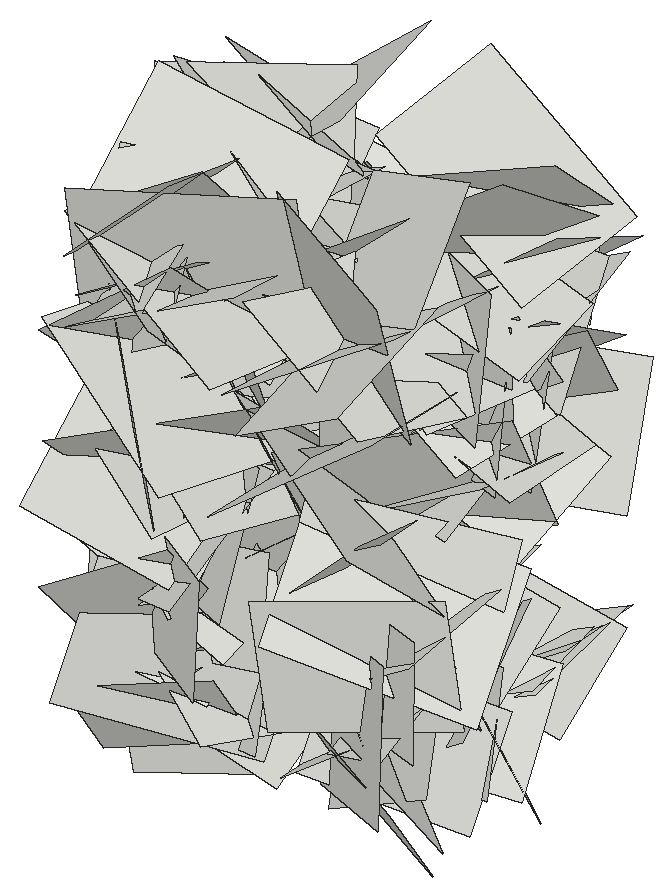
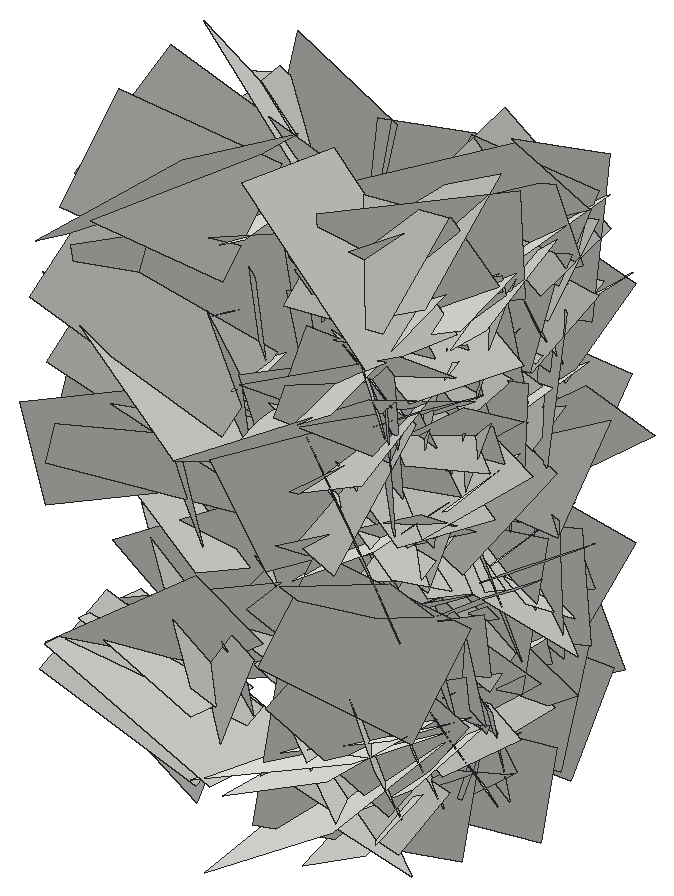
# SketchUp Ruby script. Lengths in inches.
U = 1.inch
M = Sketchup.active_model
def pt(a) = Geom::Point3d.new(a.map { |v| v * U })
def face(e, loops, mat)
  f = e.add_face(loops[0].map { |a| pt(a) })
  loops[1..].each { |l| e.add_face(l.map { |a| pt(a) }).erase! }
  f.material = f.back_material = mat if mat
  f
end
# faces: each face lists its corners as indices into pts; further lists are holes
def faces(e, pts, list, mat = nil) = list.each { |f| face(e, (f[0].is_a?(Array) ? f : [f]).map { |l| l.map { |i| pts[i] } }, mat) }
# xy, xz, yz: faces in a plane at the given z, y or x. An outline is a flat list of corners, or four numbers for a rectangle; further outlines are holes
def ring(l) = l.size == 4 ? [[l[0], l[1]], [l[2], l[1]], [l[2], l[3]], [l[0], l[3]]] : l.each_slice(2).to_a
def flat(e, list, mat, &to3) = list.each { |f| face(e, (f[0].is_a?(Array) ? f : [f]).map { |l| ring(l).map { |u, v| to3.(u, v) } }, mat) }
def xy(e, z, list, mat = nil) = flat(e, list, mat) { |x, y| [x, y, z] }
def xz(e, y, list, mat = nil) = flat(e, list, mat) { |x, z| [x, y, z] }
def yz(e, x, list, mat = nil) = flat(e, list, mat) { |y, z| [x, y, z] }
def lines(e, pts, list) = list.each { |a, b| e.add_line(pt(pts[a]), pt(pts[b])) }
# prism: a flat outline (further loops are holes) pulled along v
def prism(e, loops, v, mat = nil)
  f = face(e, loops, mat); d = Geom::Vector3d.new(v.map { |x| x * U })
  f.pushpull(f.normal.samedirection?(d) ? d.length : -d.length)
end
def box(e, o, s, mat = nil) = prism(e, [[o, [o[0] + s[0], o[1], o[2]], [o[0] + s[0], o[1] + s[1], o[2]], [o[0], o[1] + s[1], o[2]]]], [0, 0, s[2]], mat)
def at(x, y, z, deg = 0) = Geom::Transformation.translation(pt([x, y, z])) * Geom::Transformation.rotation(ORIGIN, Z_AXIS, deg.degrees)
def axes(o, x, y, z) = Geom::Transformation.new([*x, 0, *y, 0, *z, 0, *pt(o).to_a, 1])
def part(name) = M.definitions.add(name)
# library, detail: a bought-in or finely detailed component or shape, given as its bounding box
def library(name, o, s) = part(name).tap { |d| box(d.entities, o, s) }
def detail(e, o, s) = box(e.add_group.entities, o, s)
def put(e, d, t, mat = nil) = e.add_instance(d, t).tap { |i| i.material = mat if mat }
def group(e, t, mat = nil) = e.add_group.tap { |g| g.transformation = t; g.material = mat if mat }.entities
root = M.entities
c1 = part("Component\#6")
p = [[0.01,0,0],[0,3.24,4.54],[4.32,3.24,4.54],[4.33,0,0]]
faces(c1.entities,p,[[0,1,2,3]])
put(root,c1,axes([414.68,192.1875,23.6],[-0.04344,0.89705,-0.17333],[0.1764,-0.16328,-0.88435],[-0.95226,-0.07116,-0.15591]))
put(root,c1,axes([410.71,200.85,9.74],[0.02518,0.49854,0.49521],[0.19267,0.47427,-0.48618],[0.7195,-0.14445,0.11286]))
put(root,c1,axes([414.68,200.46,4.14],[-0.03987,0.66432,-0.22968],[-0.12809,-0.2327,-0.65325],[-0.73398,0.00452,0.12648]))
put(root,c1,axes([410.71,196.11,19.5625],[-0.1708,0.27531,1.11719],[-0.21419,1.10379,-0.30115],[1.2007,0.23607,0.1052]))
put(root,c1,axes([410.71,195.27,-1.16],[-0.10176,-0.07093,0.82892],[0.16666,0.81783,0.08819],[0.86597,-0.16573,0.08043]))
put(root,c1,axes([414.68,202.11,15.27],[-0.00741,-0.76642,-0.19435],[-0.02033,-0.19414,0.76626],[-0.83787,0.01149,-0.01688]))
put(root,c1,axes([414.68,201.99,11.3125],[0.07595,0.62186,-0.76254],[0.14567,-0.76339,-0.60964],[-1.03278,-0.06194,-0.14206]))
put(root,c1,axes([410.71,202.38,16.09],[-0.07402,-0.92988,-0.45649],[-0.17154,-0.44211,0.92536],[1.08456,-0.13339,0.1152]))
put(root,c1,axes([410.71,193.92,18.08],[-0.13809,0.41624,-1.10581],[-0.27382,-1.09563,-0.38198],[1.22215,-0.19844,-0.21052]))
put(root,c1,axes([414.68,193.9,23.36],[-0.05376,0.55183,-0.55937],[0.04326,-0.55793,-0.55411],[-0.83178,-0.06469,0.00734]))
put(root,c1,axes([410.71,196.25,20.97],[0.03433,0.46285,-0.75346],[-0.09275,-0.74858,-0.46362],[0.93272,-0.09148,-0.01837]))
put(root,c1,axes([410.71,193.09,19.46],[0.07295,0.25641,0.83596],[-0.12348,0.83376,-0.24615],[0.9186,0.09171,-0.09948]))
put(root,c1,axes([414.68,200.69,6.875],[0.16125,-0.91938,-0.30199],[0.04119,-0.29965,0.93182],[-1.02494,-0.15668,-0.01006]))
put(root,c1,axes([410.71,194.43,21.03],[-0.18864,1.08922,-0.2367],[-0.12278,-0.25647,-1.09312],[1.17512,0.14806,-0.15221]))
put(root,c1,axes([410.71,195.95,14.86],[-0.17446,0.9838,0.62037],[-0.19333,0.59697,-0.99508],[1.2176,0.23574,-0.06911]))
put(root,c1,axes([410.71,200.41,3.58],[-0.05776,-0.87144,-0.04483],[0.06577,-0.04867,0.87073],[0.92261,-0.05109,-0.06488]))
put(root,c1,axes([410.71,198.3125,4.47],[-0.08144,0.93817,-0.09306],[-0.01009,-0.09413,-0.94116],[0.99929,0.07551,-0.01709]))
put(root,c1,axes([410.71,200.05,13.66],[0.07814,0.81604,-0.08962],[-0.02759,-0.08761,-0.81916],[0.86976,-0.0761,-0.01794]))
put(root,c1,axes([410.71,196.375,20.79],[-0.12547,0.87042,-0.10702],[0.18806,-0.08199,-0.86307],[0.91037,0.1369,0.16354]))
put(root,c1,axes([410.71,195.73,16.63],[-0.01219,-0.78698,0.32297],[0.05977,0.32158,0.78561],[0.89973,-0.03203,-0.04781]))
put(root,c1,axes([414.68,200.82,0.59],[-0.02153,-0.73416,-0.35765],[0.0933,-0.35764,0.72915],[-0.8606,-0.02041,0.08799]))
put(root,c1,axes([410.71,193.46,10.77],[0.10152,0.90556,-0.18731],[-0.17799,-0.16815,-0.89879],[0.96391,-0.12642,-0.14624]))
put(root,c1,axes([410.71,196.17,12.88],[-0.06274,0.02618,0.84664],[0.15393,0.83645,-0.01571],[0.88457,-0.1437,0.06278]))
put(root,c1,axes([410.71,195.4375,18.11],[0.16874,-0.51977,-0.57708],[-0.05885,-0.59519,0.52076],[0.82114,0.06415,0.15591]))
put(root,c1,axes([414.68,195.9375,9.16],[-0.07841,0.69576,-0.29748],[0.09095,-0.28926,-0.69787],[-0.79692,-0.10147,-0.05038]))
put(root,c1,axes([410.71,198.67,11.97],[-0.07539,0.76068,0.50866],[0.0723,0.51318,-0.75791],[0.96729,0.02092,0.0963]))
put(root,c1,axes([414.68,195.99,4.23],[0.18601,0.0566,0.88651],[-0.05201,0.90288,-0.04793],[-0.94017,-0.03875,0.17804]))
put(root,c1,axes([414.68,197.35,3.52],[-0.03443,0.41092,0.66217],[0.08038,0.66126,-0.40665],[-0.82215,0.04744,-0.06748]))
put(root,c1,axes([410.71,192.22,20.81],[0.00161,0.62306,-0.59539],[0.0785,-0.59329,-0.62067],[0.91013,0.05007,0.05459]))
put(root,c1,axes([414.68,202.74,-0.14],[-0.03158,-0.64507,0.25861],[-0.01592,0.25938,0.64528],[-0.73651,0.02205,-0.02503]))
put(root,c1,axes([410.71,195.86,16.68],[0.06531,-0.43873,0.684],[0.07025,0.68639,0.43429],[0.8585,-0.02279,-0.08757]))
put(root,c1,axes([414.68,202.51,19.98],[-0.06792,0.48446,-0.5602],[0.10116,-0.55221,-0.48846],[-0.77852,-0.11402,-0.01459]))
put(root,c1,axes([414.68,192.04,10.01],[0.12172,0.5206,-0.6372],[-0.01939,-0.6416,-0.52749],[-0.87198,0.08694,-0.07722]))
put(root,c1,axes([414.68,198.38,4.95],[0.02223,0.32868,-0.55446],[-0.17267,-0.53404,-0.32274],[-0.66105,0.15055,0.06565]))
put(root,c1,axes([410.71,199.37,10.67],[-0.09558,-1.01864,0.46326],[-0.13943,0.47118,1.01047],[1.17795,-0.02688,0.1572]))
put(root,c1,axes([414.68,192.95,10.8],[-0.02962,0.02518,0.78508],[0.12702,0.77652,-0.02064],[-0.82287,0.11896,-0.03145]))
put(root,c1,axes([414.68,200.03,9.27],[0.00412,-0.60297,0.30435],[-0.07057,0.30253,0.60022],[-0.71247,-0.03345,-0.05769]))
put(root,c1,axes([414.68,199.6875,17.84],[-0.07891,0.44569,0.39814],[-0.07493,0.39183,-0.45185],[-0.62903,-0.10259,0.00388]))
put(root,c1,axes([414.68,200.4375,8.06],[0.17377,0.75884,-0.49804],[0.05898,-0.51355,-0.76415],[-0.96033,0.10576,-0.13705]))
put(root,c1,axes([414.68,195.68,15.75],[-0.06715,-0.51242,0.33521],[-0.05381,0.34023,0.51051],[-0.64683,0.02489,-0.07727]))
put(root,c1,axes([414.68,198.91,12.75],[0.15355,-0.10183,1.00426],[0.21738,0.99636,0.07145],[-1.04766,0.19182,0.16201]))
put(root,c1,axes([414.68,196.5625,6.92],[-0.07674,-0.09799,-0.6482],[0.03176,-0.65195,0.09521],[-0.69417,-0.019,0.07601]))
put(root,c1,axes([414.68,199.23,1.1],[0.00098,-0.71414,-0.15761],[0.04174,-0.15733,0.71311],[-0.77408,-0.00939,0.03826]))
put(root,c1,axes([414.68,192.26,20.51],[0.14395,0.6641,-0.62024],[0.10915,-0.63433,-0.65665],[-0.95701,0.02754,-0.16819]))
put(root,c1,axes([414.68,193.91,15.9375],[-0.03263,0.61645,-0.26034],[0.02336,-0.25954,-0.61716],[-0.70894,-0.03692,-0.00835]))
put(root,c1,axes([414.68,202.9,8.46],[0.28421,-0.45126,-0.90988],[0.10984,-0.92399,0.48879],[-1.07096,-0.21452,-0.19133]))
put(root,c1,axes([410.71,199.68,18.17],[-0.10811,0.81171,0.57509],[0.11351,0.5837,-0.80488],[1.04835,0.0205,0.14645]))
put(root,c1,axes([414.68,193.57,4.75],[-0.0218,0.6351,0.02763],[-0.03876,0.02642,-0.63443],[-0.67273,-0.0221,0.03566]))
put(root,c1,axes([410.71,189.31,11.46],[0.01967,0.80876,0.77653],[-0.21901,0.76581,-0.79265],[1.16812,0.12996,-0.16169]))
put(root,c1,axes([410.71,202.76,13.17],[-0.11284,-1.03894,-0.17524],[0.03066,-0.17895,1.04335],[1.11641,-0.1001,-0.04636]))
put(root,c1,axes([414.68,195.85,11.01],[0.15114,0.73817,0.19544],[-0.07767,0.21113,-0.74396],[-0.80568,0.11812,0.10838]))
put(root,c1,axes([414.68,190.79,19.57],[-0.04866,0.55121,0.30162],[-0.00575,0.30207,-0.55285],[-0.66601,-0.04288,-0.01726]))
put(root,c1,axes([410.71,196.07,8.125],[0.08332,-0.69698,-0.457],[0.10667,-0.44773,0.70016],[0.87699,0.12068,-0.04174]))
put(root,c1,axes([414.68,199.64,2.06],[0.21894,0.61345,0.59822],[-0.01858,0.61825,-0.62794],[-0.90807,0.13525,0.15708]))
put(root,c1,axes([414.68,202.56,19.21],[-0.06396,-0.26998,-0.58675],[0.04641,-0.58965,0.26682],[-0.68306,-0.01478,0.07307]))
put(root,c1,axes([410.71,197.24,20.32],[0.11105,0.4932,0.81979],[-0.10012,0.82599,-0.48487],[1.00916,0.02768,-0.13831]))
put(root,c1,axes([410.71,196.19,13.89],[-0.03711,0.95345,-0.08325],[0.1071,-0.07916,-0.94908],[1.00884,0.04348,0.09769]))
put(root,c1,axes([414.68,198.53,13.8],[0.10676,-0.41647,0.70694],[0.09382,0.7136,0.40779],[-0.86465,0.02601,0.13154]))
put(root,c1,axes([414.68,201.03,8.02],[0.03451,-0.61291,-0.20918],[-0.0475,-0.21108,0.61149],[-0.68484,-0.01625,-0.05296]))
put(root,c1,axes([414.68,199.53,17.66],[0.07108,0.22718,0.77768],[0.14032,0.76678,-0.23541],[-0.84726,0.14605,0.02626]))
put(root,c1,axes([414.68,196.1,5.28],[0.08762,-0.56519,-0.39893],[-0.0287,-0.4041,0.56691],[-0.73275,-0.05175,-0.06991]))
put(root,c1,axes([410.71,192.44,8.79],[-0.05887,1.04295,0.25043],[0.00297,0.2509,-1.04431],[1.13694,0.05335,0.0157]))
put(root,c1,axes([410.71,193.71,0.46],[0.00413,-0.52236,0.7551],[0.18121,0.74232,0.51263],[0.95624,-0.13842,-0.10041]))
put(root,c1,axes([410.71,195.28,4.79],[0.03702,0.87634,0.85063],[-0.28559,0.83554,-0.84973],[1.26267,0.16329,-0.21713]))
put(root,c1,axes([410.71,203.91,5.3125],[0.18463,-0.58129,-0.78091],[-0.13848,-0.80009,0.56643],[1.02258,-0.00339,0.2177]))
put(root,c1,axes([410.71,198.93,5.125],[0.08676,0.85287,0.14934],[0.16568,0.13299,-0.84515],[0.90272,-0.10637,0.14076]))
put(root,c1,axes([410.71,198.84,9.75],[-0.24721,-0.9594,-0.88495],[-0.06038,-0.89063,0.98057],[1.38221,-0.2105,-0.11544]))
put(root,c1,axes([410.71,202.1,18.26],[-0.1919,-1.13475,-0.09678],[0.16378,-0.12156,1.13628],[1.19604,-0.16542,-0.17113]))
put(root,c1,axes([414.68,194.11,10.49],[0.01019,-0.66626,0.06574],[0.1187,0.06642,0.65679],[-0.69967,0.00157,0.11238]))
put(root,c1,axes([410.71,200.51,5.45],[-0.07717,-0.59417,-0.91785],[0.09928,-0.91989,0.58806],[1.15472,0.03938,-0.1119]))
put(root,c1,axes([410.71,205.24,14.9],[-0.1168,-0.46047,-1.13614],[-0.0362,-1.13913,0.465],[1.29896,-0.07315,-0.0892]))
put(root,c1,axes([410.71,194.25,1.05],[0.1707,-0.55728,0.79671],[-0.04122,0.80323,0.5697],[1.02978,0.12452,-0.10926]))
put(root,c1,axes([410.71,194.35,10.5],[-0.1187,0.07765,-1.12146],[0.14385,-1.11784,-0.09095],[1.18288,0.14373,-0.10148]))
put(root,c1,axes([410.71,197.36,24.8],[-0.09794,1.0389,-0.68546],[-0.01654,-0.68826,-1.04104],[1.31923,0.0685,-0.06394]))
put(root,c1,axes([414.68,199.74,12.37],[0.13977,-0.41949,-0.41774],[-0.0557,-0.43458,0.41982],[-0.62506,-0.05508,-0.13082]))
put(root,c1,axes([414.68,199.42,15.6],[0.03605,-0.49998,-0.38134],[0.14474,-0.36691,0.49324],[-0.65063,-0.10932,0.0886]))
put(root,c1,axes([410.71,200.08,24.34],[0.03463,0.75517,-0.67877],[0.20748,-0.67107,-0.73718],[1.05612,0.10708,0.16708]))
put(root,c1,axes([410.71,199.09,16.39],[0.13116,-1.14374,0.05938],[-0.13174,0.04596,1.1443],[1.20683,0.12933,0.11846]))
put(root,c1,axes([410.71,192.66,5.0625],[0.03803,0.06475,1.02957],[0.25075,1.00223,-0.07127],[1.06436,-0.23842,-0.02]))
put(root,c1,axes([410.71,196.53,2.03],[0.14871,0.38131,0.94323],[0.09041,0.94439,-0.39446],[1.07463,-0.13222,-0.09734]))
put(root,c1,axes([410.71,200.2,14.91],[0.20407,-0.96139,-0.18597],[0.07393,-0.17559,0.97991],[1.03533,0.20204,-0.03331]))
put(root,c1,axes([410.71,198.375,11.05],[-0.00636,-0.47599,-1.14741],[-0.03555,-1.14695,0.47597],[1.31628,-0.03327,0.00731]))
put(root,c1,axes([410.71,202.25,12.93],[-0.19135,-1.27912,0.12446],[0.2118,0.09622,1.27869],[1.34571,-0.19703,-0.18355]))
put(root,c1,axes([410.71,197.86,18.23],[0.19608,0.2602,-1.0463],[-0.01915,-1.06069,-0.26697],[1.14269,-0.06243,0.17507]))
put(root,c1,axes([410.71,197.84,4.84],[0.11369,-0.36766,-0.96616],[0.19069,-0.94989,0.38144],[1.07906,0.2066,0.03439]))
put(root,c1,axes([410.71,200.375,7.61],[0.26418,-0.51362,-0.84712],[0.05211,-0.86603,0.53955],[1.04881,0.1724,0.18657]))
put(root,c1,axes([410.71,203.04,12.11],[0.14841,-0.94408,-0.5752],[0.05434,-0.57362,0.95398],[1.17058,0.14632,0.02864]))
put(root,c1,axes([410.71,199.56,18.73],[0.07364,1.07871,-0.62029],[-0.05176,-0.61841,-1.08091],[1.31797,-0.08456,-0.00779]))
put(root,c1,axes([410.71,204.42,20.53],[0.1154,-1.25003,-0.28156],[-0.14973,-0.29256,1.24425],[1.34995,0.07441,0.16208]))
put(root,c1,axes([410.71,195.93,15.54],[0.04965,0.25406,1.2028],[0.02984,1.20314,-0.25523],[1.30276,-0.03724,-0.03999]))
put(root,c1,axes([410.71,198.85,12.57],[0.15345,0.48368,1.12599],[-0.09378,1.13498,-0.47617],[1.29562,0.02486,-0.16783]))
put(root,c1,axes([410.71,200.7,5.85],[0.20906,1.0682,-0.14016],[0.07965,-0.15578,-1.08152],[1.13921,-0.18514,0.10133]))
put(root,c1,axes([410.71,194.09,6.34],[0.25898,1.07168,-0.21064],[-0.01285,-0.21318,-1.09862],[1.15764,-0.24212,0.03493]))
put(root,c1,axes([410.71,192.7,21.39],[0.08893,0.79245,0.9015],[0.06254,0.89988,-0.79652],[1.27076,-0.09974,-0.02389]))
put(root,c1,axes([410.71,199.38,-0.0625],[0.15183,-0.50198,1.07326],[0.00307,1.08122,0.50532],[1.25594,0.05804,-0.13098]))
put(root,c1,axes([410.71,200.25,4.79],[0.06637,1.27776,-0.24675],[-0.01199,-0.2465,-1.2793],[1.3794,-0.06362,0.00075]))
put(root,c1,axes([410.71,192.73,15.73],[0.12897,1.2724,-0.23633],[-0.08155,-0.22984,-1.27707],[1.36939,-0.13352,-0.05379]))
put(root,c1,axes([410.71,200.21,21.54],[0.14018,1.21556,-0.55877],[-0.14242,-0.54659,-1.22085],[1.41094,-0.17594,-0.06772]))
put(root,c1,axes([410.71,190.45,18.05],[0.16537,1.24759,-0.14593],[-0.05265,-0.14081,-1.25691],[1.33042,-0.16065,-0.0316]))
put(root,c1,axes([410.71,190.86,3.39],[0.21383,0.32739,1.20741],[-0.09698,1.22359,-0.31649],[1.32251,0.03679,-0.21843]))
put(root,c1,axes([410.71,195.52,16.87],[0.17814,-1.09516,0.21581],[0.19304,0.24222,1.08736],[1.16734,0.12707,-0.21275]))
put(root,c1,axes([410.71,201.79,17.38],[0.19939,0.73728,-1.06028],[-0.09629,-1.06126,-0.75408],[1.36551,-0.18249,0.10164]))
put(root,c1,axes([410.71,196.26,4.8],[0.10051,-0.43998,1.12809],[0.21352,1.12151,0.42048],[1.26562,-0.15427,-0.16053]))
put(root,c1,axes([410.71,191.67,21.5],[0.0579,1.33618,-0.15223],[0.05318,-0.15428,-1.33612],[1.42453,-0.04855,0.05606]))
put(root,c1,axes([410.71,198.6875,16.83],[0.02201,1.26014,0.56955],[0.0456,0.56875,-1.25994],[1.46513,-0.03663,0.03065]))
put(root,c1,axes([410.71,196.95,13.22],[0.12152,0.35472,1.26895],[0.01769,1.27325,-0.35743],[1.39654,-0.047,-0.10589]))
put(root,c1,axes([410.71,197.84,15.77],[0.08558,0.66637,-1.22765],[0.01617,-1.23004,-0.66667],[1.48057,-0.02508,0.07824]))
put(root,c1,axes([410.71,193.34,3.5],[0.3285,0.68164,0.95344],[0.04901,0.97833,-0.71446],[1.2414,-0.219,-0.22409]))
put(root,c1,axes([410.71,192.59,17.15],[0.08597,-0.32374,1.28455],[0.18245,1.27862,0.31138],[1.3923,-0.14756,-0.12012]))
put(root,c1,axes([410.71,199.09,4.9],[0.11121,1.25407,0.182],[0.25083,0.16003,-1.23904],[1.31962,-0.1361,0.22018]))
put(root,c1,axes([410.71,194.4,9.86],[0.11876,-1.04596,0.91618],[0.1474,0.92297,1.03671],[1.46651,-0.00807,-0.1784]))
put(root,c1,axes([410.71,202.95,19.72],[0.19445,-0.3512,-1.29554],[0.25274,-1.27827,0.38028],[1.40021,0.2795,0.11127]))
put(root,c1,axes([424.49,202.95,19.72],[-0.19445,-0.3512,-1.29554],[-0.25274,-1.27827,0.38028],[-1.40021,0.2795,0.11127]))
put(root,c1,axes([424.49,194.4,9.86],[-0.11876,-1.04596,0.91618],[-0.1474,0.92297,1.03671],[-1.46651,-0.00807,-0.1784]))
put(root,c1,axes([424.49,199.09,4.9],[-0.11121,1.25407,0.182],[-0.25083,0.16003,-1.23904],[-1.31962,-0.1361,0.22018]))
put(root,c1,axes([424.49,192.59,17.15],[-0.08597,-0.32374,1.28455],[-0.18245,1.27862,0.31138],[-1.3923,-0.14756,-0.12012]))
put(root,c1,axes([424.49,193.34,3.5],[-0.3285,0.68164,0.95344],[-0.04901,0.97833,-0.71446],[-1.2414,-0.219,-0.22409]))
put(root,c1,axes([424.49,197.84,15.77],[-0.08558,0.66637,-1.22765],[-0.01617,-1.23004,-0.66667],[-1.48057,-0.02508,0.07824]))
put(root,c1,axes([424.49,196.95,13.22],[-0.12152,0.35472,1.26895],[-0.01769,1.27325,-0.35743],[-1.39654,-0.047,-0.10589]))
put(root,c1,axes([424.49,198.6875,16.83],[-0.02201,1.26014,0.56955],[-0.0456,0.56875,-1.25994],[-1.46513,-0.03663,0.03065]))
put(root,c1,axes([424.49,191.67,21.5],[-0.0579,1.33618,-0.15223],[-0.05318,-0.15428,-1.33612],[-1.42453,-0.04855,0.05606]))
put(root,c1,axes([424.49,196.26,4.8],[-0.10051,-0.43998,1.12809],[-0.21352,1.12151,0.42048],[-1.26562,-0.15427,-0.16053]))
put(root,c1,axes([424.49,201.79,17.38],[-0.19939,0.73728,-1.06028],[0.09629,-1.06126,-0.75408],[-1.36551,-0.18249,0.10164]))
put(root,c1,axes([424.49,195.52,16.87],[-0.17814,-1.09516,0.21581],[-0.19304,0.24222,1.08736],[-1.16734,0.12707,-0.21275]))
put(root,c1,axes([424.49,190.86,3.39],[-0.21383,0.32739,1.20741],[0.09698,1.22359,-0.31649],[-1.32251,0.03679,-0.21843]))
put(root,c1,axes([424.49,190.45,18.05],[-0.16537,1.24759,-0.14593],[0.05265,-0.14081,-1.25691],[-1.33042,-0.16065,-0.0316]))
put(root,c1,axes([424.49,200.21,21.54],[-0.14018,1.21556,-0.55877],[0.14242,-0.54659,-1.22085],[-1.41094,-0.17594,-0.06772]))
put(root,c1,axes([424.49,192.73,15.73],[-0.12897,1.2724,-0.23633],[0.08155,-0.22984,-1.27707],[-1.36939,-0.13352,-0.05379]))
put(root,c1,axes([424.49,199.38,-0.0625],[-0.15183,-0.50198,1.07326],[-0.00307,1.08122,0.50532],[-1.25594,0.05804,-0.13098]))
put(root,c1,axes([424.49,192.7,21.39],[-0.08893,0.79245,0.9015],[-0.06254,0.89988,-0.79652],[-1.27076,-0.09974,-0.02389]))
put(root,c1,axes([424.49,194.09,6.34],[-0.25898,1.07168,-0.21064],[0.01285,-0.21318,-1.09862],[-1.15764,-0.24212,0.03493]))
put(root,c1,axes([424.49,200.7,5.85],[-0.20906,1.0682,-0.14016],[-0.07965,-0.15578,-1.08152],[-1.13921,-0.18514,0.10133]))
put(root,c1,axes([424.49,198.85,12.57],[-0.15345,0.48368,1.12599],[0.09378,1.13498,-0.47617],[-1.29562,0.02486,-0.16783]))
put(root,c1,axes([424.49,195.93,15.54],[-0.04965,0.25406,1.2028],[-0.02984,1.20314,-0.25523],[-1.30276,-0.03724,-0.03999]))
put(root,c1,axes([424.49,204.42,20.53],[-0.1154,-1.25003,-0.28156],[0.14973,-0.29256,1.24425],[-1.34995,0.07441,0.16208]))
put(root,c1,axes([424.49,199.56,18.73],[-0.07364,1.07871,-0.62029],[0.05176,-0.61841,-1.08091],[-1.31797,-0.08456,-0.00779]))
put(root,c1,axes([424.49,203.04,12.11],[-0.14841,-0.94408,-0.5752],[-0.05434,-0.57362,0.95398],[-1.17058,0.14632,0.02864]))
put(root,c1,axes([424.49,200.375,7.61],[-0.26418,-0.51362,-0.84712],[-0.05211,-0.86603,0.53955],[-1.04881,0.1724,0.18657]))
put(root,c1,axes([424.49,197.84,4.84],[-0.11369,-0.36766,-0.96616],[-0.19069,-0.94989,0.38144],[-1.07906,0.2066,0.03439]))
put(root,c1,axes([424.49,197.86,18.23],[-0.19608,0.2602,-1.0463],[0.01915,-1.06069,-0.26697],[-1.14269,-0.06243,0.17507]))
put(root,c1,axes([424.49,202.25,12.93],[0.19135,-1.27912,0.12446],[-0.2118,0.09622,1.27869],[-1.34571,-0.19703,-0.18355]))
put(root,c1,axes([424.49,198.375,11.05],[0.00636,-0.47599,-1.14741],[0.03555,-1.14695,0.47597],[-1.31628,-0.03327,0.00731]))
put(root,c1,axes([424.49,200.2,14.91],[-0.20407,-0.96139,-0.18597],[-0.07393,-0.17559,0.97991],[-1.03533,0.20204,-0.03331]))
put(root,c1,axes([424.49,196.53,2.03],[-0.14871,0.38131,0.94323],[-0.09041,0.94439,-0.39446],[-1.07463,-0.13222,-0.09734]))
put(root,c1,axes([424.49,192.66,5.0625],[-0.03803,0.06475,1.02957],[-0.25075,1.00223,-0.07127],[-1.06436,-0.23842,-0.02]))
put(root,c1,axes([424.49,199.09,16.39],[-0.13116,-1.14374,0.05938],[0.13174,0.04596,1.1443],[-1.20683,0.12933,0.11846]))
put(root,c1,axes([424.49,200.08,24.34],[-0.03463,0.75517,-0.67877],[-0.20748,-0.67107,-0.73718],[-1.05612,0.10708,0.16708]))
put(root,c1,axes([420.52,199.42,15.6],[-0.03605,-0.49998,-0.38134],[-0.14474,-0.36691,0.49324],[0.65063,-0.10932,0.0886]))
put(root,c1,axes([420.52,199.74,12.37],[-0.13977,-0.41949,-0.41774],[0.0557,-0.43458,0.41982],[0.62506,-0.05508,-0.13082]))
put(root,c1,axes([424.49,197.36,24.8],[0.09794,1.0389,-0.68546],[0.01654,-0.68826,-1.04104],[-1.31923,0.0685,-0.06394]))
put(root,c1,axes([424.49,188.68,19.83],[0.08458,1.11358,0.50301],[0.01593,0.50315,-1.11627],[-1.29513,0.07891,0.01912]))
put(root,c1,axes([424.49,194.35,10.5],[0.1187,0.07765,-1.12146],[-0.14385,-1.11784,-0.09095],[-1.18288,0.14373,-0.10148]))
put(root,c1,axes([424.49,194.25,1.05],[-0.1707,-0.55728,0.79671],[0.04122,0.80323,0.5697],[-1.02978,0.12452,-0.10926]))
put(root,c1,axes([424.49,205.24,14.9],[0.1168,-0.46047,-1.13614],[0.0362,-1.13913,0.465],[-1.29896,-0.07315,-0.0892]))
put(root,c1,axes([424.49,200.51,5.45],[0.07717,-0.59417,-0.91785],[-0.09928,-0.91989,0.58806],[-1.15472,0.03938,-0.1119]))
put(root,c1,axes([420.52,194.11,10.49],[-0.01019,-0.66626,0.06574],[-0.1187,0.06642,0.65679],[0.69967,0.00157,0.11238]))
put(root,c1,axes([424.49,202.1,18.26],[0.1919,-1.13475,-0.09678],[-0.16378,-0.12156,1.13628],[-1.19604,-0.16542,-0.17113]))
put(root,c1,axes([424.49,198.84,9.75],[0.24721,-0.9594,-0.88495],[0.06038,-0.89063,0.98057],[-1.38221,-0.2105,-0.11544]))
put(root,c1,axes([424.49,198.93,5.125],[-0.08676,0.85287,0.14934],[-0.16568,0.13299,-0.84515],[-0.90272,-0.10637,0.14076]))
put(root,c1,axes([424.49,203.91,5.3125],[-0.18463,-0.58129,-0.78091],[0.13848,-0.80009,0.56643],[-1.02258,-0.00339,0.2177]))
put(root,c1,axes([424.49,195.28,4.79],[-0.03702,0.87634,0.85063],[0.28559,0.83554,-0.84973],[-1.26267,0.16329,-0.21713]))
put(root,c1,axes([424.49,193.71,0.46],[-0.00413,-0.52236,0.7551],[-0.18121,0.74232,0.51263],[-0.95624,-0.13842,-0.10041]))
put(root,c1,axes([424.49,192.44,8.79],[0.05887,1.04295,0.25043],[-0.00297,0.2509,-1.04431],[-1.13694,0.05335,0.0157]))
put(root,c1,axes([420.52,196.1,5.28],[-0.08762,-0.56519,-0.39893],[0.0287,-0.4041,0.56691],[0.73275,-0.05175,-0.06991]))
put(root,c1,axes([420.52,199.53,17.66],[-0.07108,0.22718,0.77768],[-0.14032,0.76678,-0.23541],[0.84726,0.14605,0.02626]))
put(root,c1,axes([420.52,201.03,8.02],[-0.03451,-0.61291,-0.20918],[0.0475,-0.21108,0.61149],[0.68484,-0.01625,-0.05296]))
put(root,c1,axes([420.52,198.53,13.8],[-0.10676,-0.41647,0.70694],[-0.09382,0.7136,0.40779],[0.86465,0.02601,0.13154]))
put(root,c1,axes([424.49,196.19,13.89],[0.03711,0.95345,-0.08325],[-0.1071,-0.07916,-0.94908],[-1.00884,0.04348,0.09769]))
